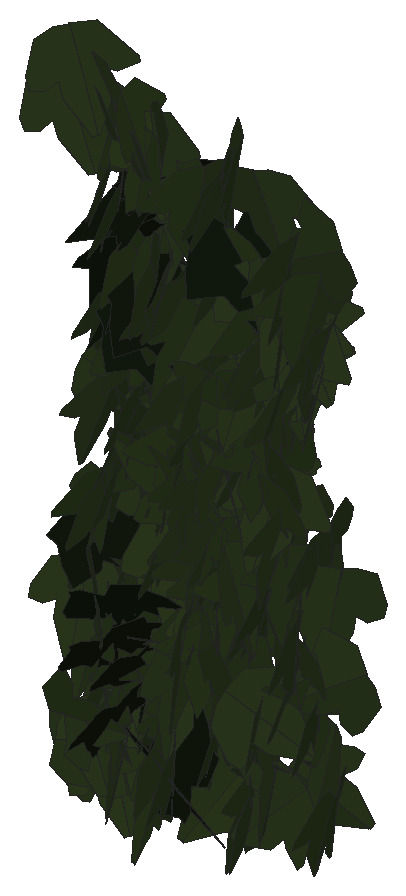
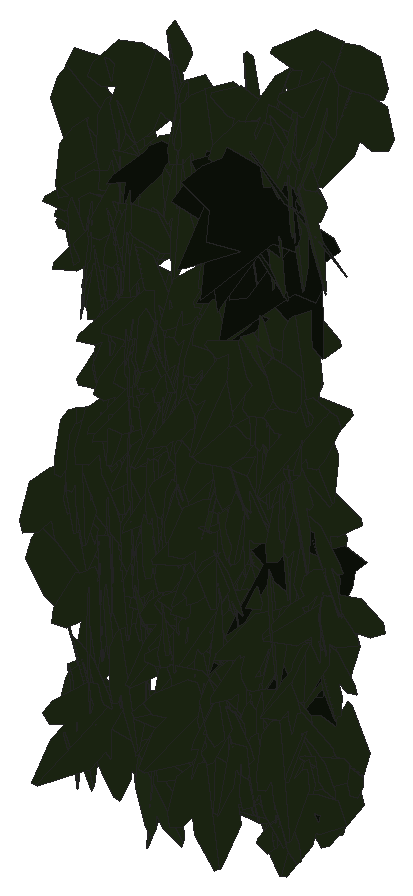
# SketchUp Ruby script. Lengths in inches.
U = 1.inch
M = Sketchup.active_model
def pt(a) = Geom::Point3d.new(a.map { |v| v * U })
def face(e, loops, mat)
  f = e.add_face(loops[0].map { |a| pt(a) })
  loops[1..].each { |l| e.add_face(l.map { |a| pt(a) }).erase! }
  f.material = f.back_material = mat if mat
  f
end
# faces: each face lists its corners as indices into pts; further lists are holes
def faces(e, pts, list, mat = nil) = list.each { |f| face(e, (f[0].is_a?(Array) ? f : [f]).map { |l| l.map { |i| pts[i] } }, mat) }
# xy, xz, yz: faces in a plane at the given z, y or x. An outline is a flat list of corners, or four numbers for a rectangle; further outlines are holes
def ring(l) = l.size == 4 ? [[l[0], l[1]], [l[2], l[1]], [l[2], l[3]], [l[0], l[3]]] : l.each_slice(2).to_a
def flat(e, list, mat, &to3) = list.each { |f| face(e, (f[0].is_a?(Array) ? f : [f]).map { |l| ring(l).map { |u, v| to3.(u, v) } }, mat) }
def xy(e, z, list, mat = nil) = flat(e, list, mat) { |x, y| [x, y, z] }
def xz(e, y, list, mat = nil) = flat(e, list, mat) { |x, z| [x, y, z] }
def yz(e, x, list, mat = nil) = flat(e, list, mat) { |y, z| [x, y, z] }
def lines(e, pts, list) = list.each { |a, b| e.add_line(pt(pts[a]), pt(pts[b])) }
# prism: a flat outline (further loops are holes) pulled along v
def prism(e, loops, v, mat = nil)
  f = face(e, loops, mat); d = Geom::Vector3d.new(v.map { |x| x * U })
  f.pushpull(f.normal.samedirection?(d) ? d.length : -d.length)
end
def box(e, o, s, mat = nil) = prism(e, [[o, [o[0] + s[0], o[1], o[2]], [o[0] + s[0], o[1] + s[1], o[2]], [o[0], o[1] + s[1], o[2]]]], [0, 0, s[2]], mat)
def at(x, y, z, deg = 0) = Geom::Transformation.translation(pt([x, y, z])) * Geom::Transformation.rotation(ORIGIN, Z_AXIS, deg.degrees)
def axes(o, x, y, z) = Geom::Transformation.new([*x, 0, *y, 0, *z, 0, *pt(o).to_a, 1])
def part(name) = M.definitions.add(name)
# library, detail: a bought-in or finely detailed component or shape, given as its bounding box
def library(name, o, s) = part(name).tap { |d| box(d.entities, o, s) }
def detail(e, o, s) = box(e.add_group.entities, o, s)
def put(e, d, t, mat = nil) = e.add_instance(d, t).tap { |i| i.material = mat if mat }
def group(e, t, mat = nil) = e.add_group.tap { |g| g.transformation = t; g.material = mat if mat }.entities
root = M.entities
M.materials.add("efeu1").color = [18, 25, 13]
M.materials.add("efeu2").color = [43, 57, 29]
c1 = part("ivyleaf_10")
p = [[0,0.5,-0.03],[-0.0625,2.02,-0.43],[-0.19,2.01,-0.46],[-0.54,1.05,-0.29],[-0.52,0.625,-0.18],[-0.83,0.76,-0.28],
  [-1.16,0.64,-0.33],[-1.15,0.33,-0.24],[-0.77,-0.39,0.02],[-0.3,-0.51,0.16],[0.04,-0.48,0.23],[-0.02,2.01,-0.4375],
  [-0.06,2.01,-0.43],[0.04,-0.49,0.23],[0.67,-0.49,0.14],[1.38,0.36,-0.2],[1.375,0.51,-0.24],[0.81,0.65,-0.19],
  [0.62,0.59,-0.15],[0.6,1.09,-0.28],[0.5,1.23,-0.31]]
faces(c1.entities,p,[[0,1,2,3,4,5,6,7,8,9,10],[11,12,0,13,14,15,16,17,18,19,20]],"efeu2")
c2 = part("ivyleaf_9")
p = [[1.54,2.16,1.25],[1.36,2.04,1.19],[-0.21,0.99,0.68],[-0.71,1.11,0.82],[-0.85,0.86,0.67],[-0.8,0.17,0.21],
  [-0.9,-0.01,0.1],[-0.67,-0.16,-0.02],[-0.08,-0.08,-0.05],[-0.03,-0.6,-0.4],[0.65,-0.88,-0.66],[0.83,-0.6,-0.49],
  [1.29,-0.42,-0.43],[1.8125,-0.07,-0.26],[1.21,0.44,0.15]]
faces(c2.entities,p,[[0,1,2,3,4,5,6,7,8,9,10,11,12,13,14]],"efeu1")
put(root,c1,axes([9.67,224.62,220.65],[0.1467,-0.41314,-0.24042],[0.0299,0.25892,-0.42669],[0.47706,0.11081,0.10067]))
put(root,c1,axes([8.58,224.6875,222.96],[0.4217,0.22163,0.15183],[0.09899,0.13451,-0.47128],[-0.24975,0.42754,0.06957]))
put(root,c1,axes([11.16,224.89,218.96],[-0.19886,-0.44425,0.11444],[0.0138,-0.13046,-0.48248],[0.45854,-0.18874,0.06415]))
put(root,c1,axes([11.23,225.09,219.62],[-0.15832,-0.24896,0.40368],[-0.07553,-0.40691,-0.28057],[0.46822,-0.14982,0.09123]))
put(root,c1,axes([9.41,224.83,221.93],[0.40818,-0.21422,0.02309],[0.03016,0.00428,-0.45145],[0.23063,0.37857,0.01817]))
put(root,c1,axes([9.81,224.63,222.27],[0.25963,-0.31984,-0.28336],[-0.10263,0.27519,-0.40465],[0.4148,0.26828,0.07725]))
put(root,c1,axes([10.75,224.69,217.39],[-0.12124,0.48435,0.02665],[-0.00457,0.02632,-0.49929],[-0.48506,-0.12131,-0.00195]))
put(root,c1,axes([9.87,224.7,214.74],[0.17093,-0.42819,-0.19347],[-0.01919,0.19935,-0.45814],[0.46948,0.16405,0.05172]))
put(root,c1,axes([8.35,224.8,214.72],[-0.10473,-0.00185,0.44101],[0.45564,0.04345,0.10053],[-0.04619,0.43282,-0.0082]))
put(root,c2,axes([9.13,224.54,216.03],[0.19407,0.39607,0.0082],[-0.01493,0.01492,-0.45191],[-0.42758,0.17925,0.0195]))
put(root,c1,axes([8.57,225,216.46],[0.1144,-0.15096,0.40973],[0.36331,-0.21494,-0.17972],[0.27501,0.34675,0.06697]))
put(root,c1,axes([8.59,224.83,216.48],[0.44025,0.14921,-0.0292],[-0.0277,-0.0116,-0.45145],[-0.16162,0.40844,-0.00216]))
put(root,c1,axes([8.47,224.71,222.43],[0.42101,0.21089,0.16816],[0.10913,0.15188,-0.46371],[-0.24666,0.42715,0.08186]))
put(root,c1,axes([10.17,224.86,221.82],[-0.17767,-0.4662,0.03308],[0.00791,-0.03838,-0.49846],[0.4673,-0.1766,0.02101]))
put(root,c2,axes([9.18,224.68,215.18],[-0.06768,0.42313,-0.08229],[0.01711,-0.07764,-0.44483],[-0.46458,-0.0645,-0.00439]))
put(root,c2,axes([9.46,224.92,214.51],[0.28678,-0.25489,0.24111],[0.18599,-0.15532,-0.38274],[0.32229,0.31644,0.00634]))
put(root,c1,axes([10.66,224.82,222.34],[0.25935,-0.42246,-0.0653],[0.00861,0.08153,-0.49323],[0.42739,0.25472,0.04957]))
put(root,c1,axes([8.68,224.88,216],[0.42862,-0.17601,0.02823],[0.02631,-0.01203,-0.45152],[0.19054,0.39762,-0.00116]))
put(root,c1,axes([11.19,224.84,218.48],[0.45715,0.17957,-0.09365],[-0.10254,0.00586,-0.48934],[-0.17464,0.46661,0.04219]))
put(root,c1,axes([10.4375,224.79,219.19],[0.13312,0.01892,-0.48158],[-0.47463,0.0919,-0.12759],[0.08369,0.49112,0.04243]))
put(root,c1,axes([11.28,224.6875,218.97],[-0.38937,0.13829,0.28155],[-0.26976,0.08139,-0.41304],[-0.16006,-0.47355,0.01123]))
put(root,c1,axes([11.65,224.94,221],[-0.15441,-0.46628,0.09347],[0.00158,-0.09878,-0.49014],[0.47556,-0.15107,0.03198]))
put(root,c1,axes([9.77,224.63,214.86],[0.0513,-0.37792,-0.32334],[0.05841,0.32738,-0.37338],[0.49392,0.00054,0.07773]))
put(root,c1,axes([11.48,224.78,216.85],[0.16866,-0.44253,-0.16036],[-0.00743,0.16782,-0.47094],[0.47064,0.16124,0.05004]))
put(root,c1,axes([11.23,225,218],[0.07446,-0.47614,0.13323],[0.02803,-0.13045,-0.48187],[0.49363,0.07923,0.00726]))
put(root,c1,axes([9.32,224.74,222.42],[-0.10805,0.41927,0.06093],[-0.00412,0.0593,-0.44816],[-0.45719,-0.09962,-0.01036]))
put(root,c1,axes([9.05,224.8,221.26],[0.16785,-0.4463,-0.15046],[-0.03289,0.14823,-0.47639],[0.46983,0.16982,0.0204]))
put(root,c1,axes([11.14,224.71,220.23],[-0.00323,-0.43689,-0.24314],[0.06248,0.24089,-0.43367],[0.49607,-0.03319,0.05303]))
put(root,c1,axes([9.9,224.91,217.93],[-0.25906,-0.00575,-0.42762],[-0.42764,-0.00034,0.25908],[-0.00327,0.49997,-0.00475]))
put(root,c1,axes([11.33,224.89,221.37],[0.0282,-0.49841,-0.02817],[-0.01488,0.02736,-0.49903],[0.49898,0.02898,-0.01329]))
put(root,c1,axes([10.76,224.82,221.03],[0.36016,-0.06913,-0.33986],[-0.31593,0.13674,-0.36262],[0.14308,0.47594,0.05482]))
put(root,c1,axes([9.93,224.96,216.17],[-0.10489,0.44599,-0.20022],[-0.06066,-0.21507,-0.44729],[-0.4851,-0.06954,0.09922]))
put(root,c2,axes([9.45,224.97,220.6],[-0.40958,0.14432,-0.16302],[0.14369,-0.08956,-0.42053],[-0.17974,-0.40047,0.0353]))
put(root,c1,axes([10.97,224.59,215.86],[0.11812,0.31878,0.36665],[0.13332,0.34158,-0.33993],[-0.4672,0.17806,-0.00431]))
put(root,c2,axes([9.06,224.66,216.47],[0.34382,0.29054,-0.06122],[-0.05464,-0.03186,-0.44811],[-0.31546,0.32218,0.0109]))
put(root,c1,axes([11.1,224.8,218.42],[-0.47018,0.16933,0.016],[-0.02026,-0.00905,-0.49951],[-0.16888,-0.47037,0.01537]))
put(root,c2,axes([9.38,224.86,221.42],[-0.39068,0.24019,0.027],[-0.02653,0.00993,-0.45156],[-0.25957,-0.36254,0.00552]))
put(root,c1,axes([11.02,224.86,222.03],[-0.48749,-0.01376,-0.1103],[0.11109,-0.0442,-0.48549],[0.00361,-0.49785,0.04615]))
put(root,c1,axes([9.32,224.74,220.8125],[0.02656,-0.42828,-0.25665],[0.08787,0.25701,-0.41979],[0.4915,-0.02281,0.08892]))
put(root,c1,axes([11.9,224.88,221.56],[-0.2256,0.00204,0.44621],[-0.44309,-0.06012,-0.22374],[0.05274,-0.49637,0.02893]))
put(root,c1,axes([10.84,224.81,219.3125],[-0.28334,0.4119,0.00766],[-0.00526,0.00568,-0.49994],[-0.41194,-0.28339,0.00111]))
put(root,c1,axes([9.65,224.95,220.21],[0.01957,-0.49961,-0.00229],[-0.00005,0.00229,-0.49999],[0.49962,0.01957,0.00004]))
put(root,c2,axes([10.6,224.92,221.28],[0.06536,-0.43431,-0.23897],[0.02007,0.24315,-0.43643],[0.4953,0.04746,0.04922]))
put(root,c1,axes([10.54,224.85,218.58],[-0.49791,-0.03979,0.0225],[-0.02257,-0.00004,-0.49949],[0.03976,-0.49841,-0.00175]))
put(root,c1,axes([9.1875,224.83,222.08],[-0.35383,0.28611,0.00606],[-0.00704,0.00139,-0.45235],[-0.30898,-0.32767,0.00337]))
put(root,c1,axes([9.85,224.99,215.81],[0.16279,0.44535,-0.15863],[-0.05178,-0.14997,-0.47416],[-0.46991,0.17081,-0.00271]))
put(root,c1,axes([11.33,224.85,221.03],[0.22017,-0.4247,-0.14543],[0.01107,0.16707,-0.47113],[0.44878,0.20424,0.08297]))
put(root,c1,axes([10.39,224.87,221.86],[0.08347,-0.47543,-0.13037],[0.00495,0.13303,-0.48195],[0.49296,0.07917,0.02692]))
put(root,c1,axes([11.17,224.95,219.91],[0.01952,-0.49885,-0.02769],[0.00394,0.02786,-0.49921],[0.4996,0.01927,0.00502]))
put(root,c1,axes([9.42,224.93,222.1],[0.44369,0.04104,0.14247],[0.14324,0.04652,-0.42814],[-0.05776,0.43055,0.03268]))
put(root,c1,axes([10.32,224.82,216.23],[-0.2992,0.10595,0.38633],[-0.38576,0.05383,-0.31352],[-0.10803,-0.48567,0.04953]))
put(root,c1,axes([9.98,224.88,219.27],[-0.1077,-0.47323,-0.12021],[0.0258,0.11741,-0.48533],[0.48758,-0.11075,-0.00087]))
put(root,c1,axes([10.36,224.89,215.3],[0.22481,-0.4226,-0.14446],[-0.03424,0.14495,-0.4773],[0.4453,0.2245,0.03623]))
put(root,c1,axes([11.07,224.89,220.48],[-0.23593,-0.42617,-0.11276],[0.07263,0.08857,-0.4867],[0.43481,-0.24604,0.02011]))
put(root,c1,axes([11.34,224.93,219.57],[-0.0264,-0.49346,-0.07616],[0.02181,0.07506,-0.49385],[0.49883,-0.0294,0.01756]))
put(root,c1,axes([10.62,225.24,217.89],[-0.00156,-0.35951,0.34749],[-0.00496,-0.34747,-0.3595],[0.49997,-0.00457,-0.00248]))
put(root,c1,axes([10.8,225.26,214.71],[0.04452,-0.13242,0.48009],[0.33447,-0.34916,-0.12733],[0.36898,0.33249,0.05749]))
put(root,c1,axes([11.38,224.99,220.3],[0.47165,0.13662,-0.09426],[-0.09351,-0.01588,-0.49092],[-0.13713,0.48071,0.01057]))
put(root,c2,axes([10.1,224.74,214.58],[-0.10758,0.11868,0.47365],[-0.28732,0.37677,-0.15967],[-0.39481,-0.30653,-0.01287]))
put(root,c1,axes([9.62,224.91,220.52],[0.27513,-0.38869,-0.1524],[-0.05347,0.14821,-0.47453],[0.41406,0.27741,0.03999]))
put(root,c1,axes([8.67,224.9,222.69],[-0.40677,0.21341,-0.04444],[0.03624,-0.02745,-0.45015],[-0.23225,-0.37806,0.0076]))
put(root,c1,axes([10.51,225.06,219.38],[-0.13753,-0.47132,0.09456],[-0.01315,-0.09463,-0.49079],[0.48053,-0.13748,0.01363]))
put(root,c1,axes([11.09,224.87,220.15],[-0.06522,-0.46595,-0.16923],[0.03089,0.16654,-0.47044],[0.49476,-0.07182,0.00707]))
put(root,c1,axes([11,224.92,220.86],[0.42008,0.26202,0.06984],[0.04411,0.06102,-0.4943],[-0.26755,0.42145,0.02815]))
put(root,c1,axes([8.73,225.08,218.6875],[-0.01959,-0.42117,0.11159],[-0.01071,-0.10696,-0.43839],[0.46927,-0.02002,-0.00535]))
put(root,c2,axes([9.17,224.96,220.71],[0.00123,0.35173,-0.26619],[0.00254,-0.25595,-0.36579],[-0.46979,-0.00047,-0.00268]))
put(root,c1,axes([9.26,225.09,218.77],[0.19305,-0.3835,0.10502],[0.05187,-0.08902,-0.44],[0.42515,0.185,0.00599]))
put(root,c1,axes([10.3,224.81,219.42],[0.03069,-0.42511,-0.26141],[0.04868,0.26321,-0.42232],[0.49668,0.00047,0.05755]))
put(root,c2,axes([9.47,224.66,216.13],[0.4351,0.15995,0.03799],[-0.0471,0.19778,-0.40037],[-0.17082,0.35288,0.20718]))
put(root,c1,axes([10.35,225.06,216.17],[-0.35039,-0.32706,0.14233],[-0.07012,-0.13246,-0.47701],[0.34973,-0.35424,0.04696]))
put(root,c2,axes([9.47,224.92,220.29],[0.10809,-0.38779,-0.29654],[-0.0523,0.29278,-0.40193],[0.48537,0.11791,0.02273]))
put(root,c1,axes([10,225.05,220],[0.24252,0.37749,-0.22064],[-0.21104,-0.11992,-0.43713],[-0.38295,0.30515,0.10116]))
put(root,c1,axes([9.91,225.05,218.43],[-0.36783,-0.32118,0.10745],[-0.03799,-0.11851,-0.48426],[0.33654,-0.36442,0.06278]))
put(root,c1,axes([8.66,224.99,217.42],[0.35257,-0.26935,-0.10453],[-0.08449,0.06311,-0.44016],[0.29877,0.3357,-0.00113]))
put(root,c1,axes([8.7,225.09,214.93],[0.38472,-0.14413,0.21202],[0.20472,-0.07504,-0.39964],[0.17549,0.40351,0.00141]))
put(root,c1,axes([10.93,224.98,217.07],[0.15772,-0.46463,-0.09613],[-0.03398,0.08998,-0.49066],[0.47325,0.16131,-0.0032]))
put(root,c1,axes([10.46,224.93,218.62],[-0.25161,0.43038,-0.03831],[0.01129,-0.03776,-0.49844],[-0.43193,-0.25169,0.00929]))
put(root,c1,axes([9.87,224.93,220.38],[0.00387,-0.47826,-0.14577],[0.03989,0.1456,-0.47666],[0.49839,-0.00793,0.03928]))
put(root,c1,axes([10.64,225.18,217.05],[-0.13861,-0.44187,0.18851],[0.02481,-0.20253,-0.45647],[0.47976,-0.11719,0.07807]))
put(root,c1,axes([10.4,224.88,221.82],[0.09556,-0.43672,-0.22393],[0.00935,0.22971,-0.44401],[0.49069,0.08067,0.05207]))
put(root,c1,axes([11.63,225.08,220.28],[0.10019,-0.4897,0.0124],[0.01504,-0.00958,-0.49968],[0.48963,0.10049,0.01281]))
put(root,c1,axes([9.9,225.14,218.66],[0.1991,-0.45163,0.07994],[0.02198,-0.07765,-0.49344],[0.45812,0.2,-0.01106]))
put(root,c1,axes([9.34,225.1,214.11],[0.36834,-0.26811,0.0332],[0.01916,-0.02907,-0.45101],[0.29098,0.34131,-0.01233]))
put(root,c1,axes([10.8125,224.98,218.71],[0.0562,-0.48016,-0.12763],[-0.00895,0.12745,-0.4834],[0.49675,0.05662,0.00573]))
put(root,c1,axes([9.48,225.05,221.17],[-0.46467,-0.06381,0.00638],[0.00847,-0.09371,-0.4417],[0.06871,-0.41997,0.09759]))
put(root,c1,axes([10.91,224.92,215.68],[0.23022,-0.39661,-0.19925],[-0.01075,0.21941,-0.44916],[0.44372,0.21109,0.0925]))
put(root,c1,axes([8.68,224.95,222.33],[-0.33006,0.30955,-0.00139],[0.00092,-0.00104,-0.4524],[-0.33432,-0.30562,0.00013]))
put(root,c1,axes([10.46,224.91,220.91],[0.07881,-0.44249,-0.21906],[0.00344,0.22232,-0.44784],[0.49374,0.06909,0.03809]))
put(root,c1,axes([10.62,225.06,218.71],[0.49853,-0.00113,-0.03825],[-0.03813,0.02777,-0.49777],[0.00325,0.49923,0.0276]))
put(root,c1,axes([11.24,224.89,220.5],[0.25227,-0.35493,-0.24574],[-0.04163,0.26329,-0.42302],[0.42968,0.23389,0.10329]))
put(root,c1,axes([8.7,225.35,214.27],[0.07627,-0.15157,0.47033],[0.31717,-0.34991,-0.1642],[0.37892,0.3234,0.04277]))
put(root,c2,axes([9.21,225.05,219.77],[0.11856,-0.37666,-0.1954],[0.00218,0.19463,-0.40458],[0.45459,0.09731,0.0529]))
put(root,c1,axes([11.33,225.07,220.25],[0.32131,-0.38017,-0.04726],[0.00173,0.06311,-0.496],[0.38309,0.31857,0.04187]))
put(root,c1,axes([8.76,224.94,217.55],[0.02758,-0.45293,-0.20999],[0.04231,0.21168,-0.451],[0.49744,0.00711,0.05001]))
put(root,c1,axes([10.05,225.16,218.1],[0.0083,-0.49268,0.08482],[-0.0046,-0.0849,-0.49272],[0.49991,0.0074,-0.00594]))
put(root,c1,axes([8.6875,225.08,221.32],[0.22037,-0.3813,-0.04882],[-0.02491,0.0409,-0.44976],[0.41416,0.20534,-0.00108]))
put(root,c1,axes([8.76,225.0625,217.65],[-0.12122,-0.48365,-0.03731],[0.00225,0.0379,-0.49856],[0.48508,-0.12104,-0.00702]))
put(root,c1,axes([10.13,225.24,217.37],[0.04746,-0.46527,0.17685],[0.04298,-0.17315,-0.46709],[0.49588,0.05954,0.02356]))
put(root,c1,axes([11.33,225.18,217.47],[-0.18455,-0.44933,0.1185],[0.00168,-0.12814,-0.4833],[0.46469,-0.17799,0.04881]))
put(root,c1,axes([11.56,225.05,219.8],[0.29363,-0.38793,-0.11529],[-0.0382,0.11523,-0.48504],[0.40289,0.29366,0.03803]))
put(root,c1,axes([9.95,225.2,218.06],[-0.06103,-0.48292,0.11431],[-0.00805,-0.11419,-0.48672],[0.4962,-0.06125,0.00617]))
put(root,c1,axes([10.83,225.15,218.99],[0.41401,-0.2799,-0.01576],[-0.01987,-0.00127,-0.4996],[0.27964,0.41431,-0.01218]))
put(root,c1,axes([9.86,225.25,215.37],[-0.05411,-0.46459,0.17672],[0.01816,-0.17949,-0.46632],[0.49673,-0.04404,0.03629]))
put(root,c1,axes([9.25,224.97,219.78],[0.41457,0.09497,0.18851],[0.14433,0.17545,-0.38994],[-0.16737,0.38655,0.13067]))
put(root,c1,axes([11.4,224.9375,220.52],[0.21001,0.42244,0.16564],[0.07592,0.14724,-0.47176],[-0.44736,0.2233,-0.0023]))
put(root,c1,axes([11.2,225.07,220.32],[0.45451,0.19228,0.08033],[0.06907,0.04285,-0.49335],[-0.19661,0.45956,0.01239]))
put(root,c1,axes([10.74,225.15,219.33],[-0.25563,0.35311,-0.24488],[0.14846,-0.19482,-0.4359],[-0.40326,-0.29556,-0.00524]))
put(root,c1,axes([9.37,225.04,219.92],[-0.37161,-0.21391,-0.16469],[0.1775,0.0328,-0.41748],[0.22608,-0.37735,0.05706]))
put(root,c1,axes([10.01,225.37,216.73],[0.11095,-0.11627,0.47347],[0.36397,-0.30331,-0.15977],[0.32437,0.38011,0.01734]))
put(root,c1,axes([10.99,225.11,219.37],[-0.30399,0.38321,-0.10364],[-0.00412,-0.13357,-0.48181],[-0.39696,-0.29207,0.08436]))
put(root,c1,axes([9.27,225.03,221.82],[-0.4263,-0.15261,-0.10466],[0.10175,0.03539,-0.44013],[0.16919,-0.40581,0.00097]))
put(root,c1,axes([9.99,225.09,215.69],[-0.3942,0.27762,-0.13242],[0.10374,-0.08263,-0.48209],[-0.28956,-0.40755,0.00754]))
put(root,c1,axes([8.73,225.09,216.1875],[0.15654,-0.03818,0.4247],[0.43324,0.1034,-0.13802],[-0.09225,0.4208,0.07245]))
put(root,c1,axes([10.52,225.24,218.03],[0.11933,0.4328,-0.22011],[-0.05,-0.2145,-0.44888],[-0.48297,0.12914,-0.00792]))
put(root,c2,axes([9.29,224.92,215.74],[0.06299,0.43016,-0.02915],[-0.01975,-0.02579,-0.4512],[-0.46514,0.05935,0.01521]))
put(root,c1,axes([9.17,225.16,220.81],[-0.39913,0.21075,-0.09436],[0.0228,-0.14005,-0.42775],[-0.24676,-0.35383,0.1131]))
put(root,c1,axes([9.45,225.33,218.16],[0.22562,-0.26815,0.2823],[0.19677,-0.20179,-0.35315],[0.36206,0.27677,0.01602]))
put(root,c1,axes([11.29,224.98,219.8],[0.10205,-0.40879,-0.26921],[-0.04827,0.26525,-0.42108],[0.48709,0.11194,0.01467]))
put(root,c1,axes([8.72,225.11,216.49],[-0.45054,-0.1109,0.05598],[-0.0558,-0.01517,-0.44892],[0.12088,-0.42035,0.00143]))
put(root,c1,axes([11.25,225.06,220.0625],[0.16661,0.46931,0.04458],[-0.02066,0.0545,-0.49659],[-0.47097,0.16363,0.03755]))
put(root,c1,axes([9.61,225.16,217.1],[0.47071,0.16678,0.02484],[0.02051,0.01649,-0.49931],[-0.16737,0.47108,0.00868]))
put(root,c1,axes([11.91,225.23,216.23],[-0.25781,0.01477,0.42815],[-0.40317,-0.17733,-0.23665],[0.14486,-0.46726,0.10335]))
put(root,c1,axes([8.47,224.93,214.44],[-0.02515,-0.1388,-0.47969],[0.42581,0.24495,-0.0932],[0.26087,-0.4132,0.10588]))
put(root,c1,axes([9.15,225.09,219.46],[-0.28321,-0.30945,-0.16346],[0.15551,0.08224,-0.41824],[0.34106,-0.29446,0.05497]))
put(root,c1,axes([11.29,225.11,215.86],[-0.35186,-0.34741,-0.07416],[0.04698,0.05795,-0.4944],[0.35212,-0.35489,-0.00814]))
put(root,c1,axes([9,225.375,215.32],[-0.0575,-0.43776,0.23464],[0.02108,-0.23815,-0.43914],[0.49624,-0.0406,0.04584]))
put(root,c1,axes([11.11,225.16,214.53],[0.36662,-0.11014,-0.32165],[-0.30949,0.0877,-0.38278],[0.14074,0.47977,-0.00387]))
put(root,c1,axes([10.42,224.89,218.49],[-0.0319,-0.29818,-0.40009],[0.12967,0.38218,-0.29517],[0.48184,-0.1226,0.05295]))
put(root,c2,axes([9.13,224.89,220.69],[0.28658,0.33495,0.08463],[0.05405,0.06417,-0.44441],[-0.36832,0.27003,0.00063]))
put(root,c1,axes([10.8125,225.11,219.85],[0.36159,-0.28896,-0.18908],[-0.10623,0.16741,-0.45901],[0.32858,0.37212,0.05968]))
put(root,c1,axes([10.35,225.26,218.33],[-0.42173,-0.09421,-0.25153],[-0.2478,-0.04416,0.43202],[-0.10362,0.48905,-0.00944]))
put(root,c1,axes([9.57,225.0625,217.23],[0.10819,-0.43754,-0.21646],[-0.03271,0.21472,-0.45036],[0.48706,0.11161,0.01784]))
put(root,c1,axes([10.59,225.18,218.45],[-0.49959,-0.01872,-0.0078],[0.01114,-0.0926,-0.49122],[0.01694,-0.49099,0.09294]))
put(root,c1,axes([8.7,225.17,219.8125],[0.02934,-0.42918,-0.06813],[-0.00865,0.06513,-0.44722],[0.4688,0.02806,-0.00399]))
put(root,c2,axes([8.65,225,217.17],[0.02937,-0.16575,-0.41731],[0.04995,0.40087,-0.16895],[0.46621,-0.03251,0.0444]))
put(root,c1,axes([11.1,225.19,218.03],[-0.20472,-0.45605,-0.01028],[0.00312,0.00987,-0.49989],[0.45616,-0.20474,-0.00119]))
put(root,c1,axes([9.15,225.1,219.4],[-0.0492,-0.39844,-0.17524],[0.06392,0.1621,-0.41528],[0.46282,-0.06475,0.03872]))
put(root,c1,axes([9.63,225.38,214.96],[-0.05239,-0.45571,0.19895],[0.00551,-0.20057,-0.45798],[0.49722,-0.04579,0.02604]))
put(root,c1,axes([9.13,225.1,218.79],[0.08411,-0.4537,-0.19258],[-0.01731,0.19252,-0.46112],[0.49257,0.08423,0.01668]))
put(root,c1,axes([8.89,225.11,217.8],[0.13103,-0.44424,-0.18837],[-0.02275,0.18929,-0.46223],[0.48199,0.1297,0.02939]))
put(root,c1,axes([9.39,225.2,220.2],[0.41446,0.18581,-0.08963],[-0.11192,0.01826,-0.43896],[-0.19081,0.3929,0.06279]))
put(root,c1,axes([10.82,225.13,218.52],[-0.44387,0.22852,-0.02764],[0.019,-0.02346,-0.49909],[-0.2294,-0.44411,0.01214]))
put(root,c1,axes([10.27,225.16,216.45],[-0.24452,-0.41841,-0.12304],[0.11736,0.07272,-0.48056],[0.42004,-0.2639,0.06265]))
put(root,c1,axes([11.24,225.1,216.48],[-0.41461,0.11529,0.25458],[-0.25037,0.04914,-0.43],[-0.12417,-0.48404,0.01698]))
put(root,c1,axes([9.83,225.3,215.76],[0.0009,-0.49762,0.0487],[-0.00581,-0.0487,-0.49759],[0.49997,0.00033,-0.00587]))
put(root,c1,axes([9.64,225.5,215.44],[-0.11029,-0.32573,0.36295],[-0.05441,-0.36158,-0.34103],[0.48464,-0.11472,0.04431]))
put(root,c1,axes([9.96,225.1875,217.46],[-0.1547,-0.46892,-0.07862],[0.02445,0.07473,-0.49378],[0.47484,-0.15662,-0.00019]))
put(root,c1,axes([9.4,225.07,220.58],[0.03823,0.41081,0.14413],[-0.06439,0.14234,-0.42298],[-0.46379,0.0141,0.07061]))
put(root,c1,axes([9.36,225.21,219.18],[-0.08718,0.42449,-0.05214],[0.00376,-0.05036,-0.44934],[-0.46162,-0.08058,0.00619]))
put(root,c1,axes([10.91,225.16,219.09],[0.14768,-0.4434,-0.17773],[-0.00121,0.18569,-0.46424],[0.47769,0.13755,0.05377]))
put(root,c1,axes([8.7,225.18,214.23],[0.3373,0.28694,0.10055],[0.07099,0.07133,-0.44101],[-0.31921,0.31906,0.00817]))
put(root,c1,axes([10.35,225.18,218.92],[-0.44313,-0.2106,-0.09636],[0.09067,0.03366,-0.49056],[0.21311,-0.45223,0.00836]))
put(root,c1,axes([10.52,225.09,219.45],[0.23048,0.42904,0.11315],[-0.05883,0.15592,-0.47141],[-0.43979,0.20399,0.12236]))
put(root,c2,axes([9.54,225.02,221.21],[0.19335,0.39618,-0.01525],[-0.00883,-0.0124,-0.45214],[-0.42808,0.1792,0.00244]))
put(root,c1,axes([9.69,225.18,215.91],[-0.03867,-0.47595,-0.14824],[0.00355,0.14842,-0.47745],[0.49849,-0.03798,-0.0081]))
put(root,c1,axes([11.56,225.3,214.62],[0.11577,-0.48569,-0.0265],[-0.00458,0.02615,-0.49929],[0.48639,0.11585,0.00161]))
put(root,c1,axes([9.4,225.28,217.54],[0.45922,0.0671,-0.06517],[-0.07289,0.02719,-0.44603],[-0.06721,0.42893,0.03846]))
put(root,c1,axes([11.48,225.16,220.25],[0.2325,-0.40137,-0.18666],[0.02558,0.22267,-0.44695],[0.44191,0.19828,0.12408]))
put(root,c1,axes([8.89,225.16,218.56],[-0.38173,0.23169,0.10717],[-0.09478,0.05408,-0.43951],[-0.25693,-0.36417,0.00291]))
put(root,c1,axes([9.61,225.27,216.17],[-0.3358,-0.36972,-0.0234],[0.0361,-0.00123,-0.49869],[0.36869,-0.33661,0.02752]))
put(root,c1,axes([8.78,225.12,214.875],[-0.2511,0.33931,0.1472],[-0.08649,0.11671,-0.42778],[-0.38753,-0.24591,0.00009]))
put(root,c1,axes([10.62,225.22,218.35],[0.13717,0.48065,0.01281],[-0.00658,0.0152,-0.49973],[-0.48077,0.13692,0.01049]))
put(root,c1,axes([9.97,225.35,217.05],[-0.17237,-0.46517,0.06245],[-0.03055,-0.05527,-0.496],[0.46835,-0.17481,-0.00937]))
put(root,c1,axes([9.9375,225.35,216.71],[0.44306,0.12122,-0.19749],[-0.193,-0.0428,-0.45926],[-0.12825,0.48319,0.00887]))
put(root,c1,axes([9.33,225.32,215.05],[0.18475,-0.46196,-0.04963],[-0.01193,0.04867,-0.49748],[0.46446,0.18501,0.00697]))
put(root,c1,axes([9.96,225.25,217.82],[-0.4854,0.06406,0.10142],[-0.10617,-0.03264,-0.48751],[-0.05583,-0.4948,0.04529]))
put(root,c1,axes([10.72,225.22,218.42],[0.0876,0.49173,0.02292],[0.01039,0.02143,-0.49943],[-0.49216,0.08798,-0.00646]))
put(root,c1,axes([9.37,225.26,219.85],[-0.41888,-0.19673,0.01003],[-0.0119,0.0004,-0.45225],[0.21239,-0.38797,-0.00556]))
put(root,c1,axes([10,225.24,218.58],[0.02836,0.49911,-0.0093],[-0.00004,-0.00931,-0.49991],[-0.4992,0.02836,-0.00049]))
put(root,c1,axes([10.96,225.14,219.29],[0.03348,0.47999,0.13596],[0.00919,0.13565,-0.48116],[-0.49879,0.03472,0.00026]))
put(root,c1,axes([9.32,225.44,218.34],[-0.04633,-0.40769,0.15134],[-0.00917,-0.14541,-0.42629],[0.46742,-0.04326,0.00664]))
put(root,c1,axes([8.71,225.25,218.1],[0.17447,-0.37345,-0.15999],[-0.06945,0.13979,-0.42315],[0.43064,0.17384,-0.00343]))
put(root,c1,axes([10.33,225.29,217.58],[0.00562,0.49445,-0.07406],[-0.00292,-0.07403,-0.49448],[-0.49996,0.00599,0.00206]))
put(root,c1,axes([8.52,224.98,216.66],[-0.02887,-0.05689,-0.44765],[0.16116,0.40377,-0.06514],[0.44035,-0.15151,-0.00551]))
put(root,c1,axes([10.19,225.28,217.4],[0.06378,-0.48544,-0.10141],[0.00979,0.10346,-0.48908],[0.49582,0.0604,0.0227]))
put(root,c1,axes([10.24,225.35,214.43],[0.41914,0.09034,-0.25722],[-0.25876,-0.01667,-0.42751],[-0.08582,0.49149,0.03277]))
put(root,c1,axes([11.44,225.39,215.1875],[0.41412,-0.27781,0.0364],[0.03686,-0.01038,-0.49853],[0.27775,0.41559,0.01188]))
put(root,c1,axes([9.66,225.34,218.68],[0.46383,0.05532,-0.04308],[-0.04604,0.00687,-0.45017],[-0.05874,0.43141,0.01269]))
put(root,c1,axes([9.42,225.41,217.68],[0.10659,-0.4186,0.06787],[0.03769,-0.05875,-0.44678],[0.45599,0.10271,0.02106]))
put(root,c1,axes([11.58,225.42,217.15],[-0.33178,-0.36029,0.10054],[0.01273,-0.14519,-0.47829],[0.37384,-0.31482,0.10552]))
put(root,c1,axes([9.375,225.36,215.59],[-0.44083,0.14657,-0.18491],[0.14391,-0.14349,-0.45684],[-0.18698,-0.45599,0.08432]))
put(root,c1,axes([9.96,225.31,216.41],[-0.41526,-0.2783,0.01063],[-0.009,-0.00567,-0.49989],[0.27835,-0.41535,-0.0003]))
put(root,c1,axes([8.78,225.23,214.01],[0.04982,0.42976,-0.05095],[-0.01763,0.05096,0.44896],[0.46682,-0.04394,0.02239]))
put(root,c1,axes([9.3,225.33,219.29],[0.12122,0.41543,-0.06613],[-0.06454,-0.04937,-0.44516],[-0.44928,0.11918,0.0461]))
put(root,c1,axes([10.76,225.19,218.7],[-0.19689,-0.39651,-0.23241],[0.09206,0.21368,-0.44256],[0.45029,-0.21706,-0.01114]))
put(root,c1,axes([9.48,225.28,219.35],[-0.0885,0.42696,0.01515],[-0.02014,0.01125,-0.45183],[-0.46095,-0.08247,0.01683]))
put(root,c1,axes([10.56,225.16,214.26],[0.13863,-0.36904,-0.30756],[-0.03331,0.31195,-0.38933],[0.47924,0.12844,0.06191]))
put(root,c1,axes([11.0625,225.33,215.83],[0.17678,-0.45679,-0.10046],[-0.00923,0.10397,-0.48898],[0.46762,0.17474,0.02832]))
put(root,c1,axes([10.31,225.29,217.66],[-0.45366,0.04093,0.2062],[-0.20743,-0.00746,-0.45488],[-0.03416,-0.49827,0.02374]))
put(root,c1,axes([9.23,225.32,218.01],[-0.169,-0.39002,-0.11685],[0.10373,0.08142,-0.43303],[0.4259,-0.17459,0.0591]))
put(root,c1,axes([9.83,225.3125,216.82],[0.22471,-0.41758,-0.15854],[-0.02545,0.16521,-0.47123],[0.44594,0.21985,0.05299]))
put(root,c1,axes([9.33,225.42,215.59],[-0.18388,-0.4629,0.04367],[-0.02632,-0.03653,-0.49797],[0.46421,-0.18543,-0.01093]))
put(root,c1,axes([9.16,225.25,214.68],[0.27635,-0.2391,-0.26836],[-0.14298,0.23017,-0.35834],[0.35199,0.28121,0.06514]))
put(root,c1,axes([11.61,225.3,214.68],[0.23985,-0.40056,-0.17897],[-0.03669,0.18494,-0.46309],[0.43718,0.23527,0.05933]))
put(root,c1,axes([11.375,225.27,215.65],[0.1697,-0.41861,-0.21441],[-0.02572,0.21933,-0.44859],[0.46962,0.16328,0.0529]))
put(root,c1,axes([9.4,225.29,218.3],[-0.34702,-0.12961,-0.27355],[0.27369,0.07357,-0.35966],[0.15933,-0.40867,0.02201]))
put(root,c1,axes([10.46,225.35,217.63],[0.14178,-0.46439,-0.11934],[-0.00035,0.12435,-0.48429],[0.47948,0.13741,0.03494]))
put(root,c1,axes([11.43,225.34,217.64],[0.07631,-0.47454,-0.1378],[0.00095,0.13957,-0.48012],[0.49414,0.07301,0.0222]))
put(root,c1,axes([10.17,225.4,216.81],[-0.32564,-0.3794,0.00343],[0.00313,-0.00721,-0.49994],[0.3794,-0.32558,0.00707]))
put(root,c1,axes([9.84,225.47,216.25],[-0.15096,-0.4745,0.0454],[0.02941,-0.05681,-0.49589],[0.47576,-0.14705,0.04506]))
put(root,c1,axes([10.1875,225.27,217.3],[0.28822,-0.21508,-0.34737],[-0.23383,0.26177,-0.35609],[0.33504,0.36772,0.05031]))
put(root,c1,axes([9.65,225.34,216.86],[-0.49785,0.03744,0.02721],[-0.02731,-0.00028,-0.49925],[-0.03737,-0.4986,0.00233]))
put(root,c2,axes([9.27,225.07,221.28],[0.31807,0.26566,0.1858],[0.0593,0.19723,-0.39916],[-0.34063,0.2824,0.104]))
put(root,c1,axes([10.39,225.43,217.08],[0.10388,-0.48619,-0.05319],[-0.00973,0.05231,-0.49716],[0.48899,0.10432,0.00141]))
put(root,c1,axes([10.34,225.6,214.26],[0.14338,-0.44437,0.17882],[0.05406,-0.17046,-0.46693],[0.47594,0.15324,-0.00084]))
put(root,c1,axes([9.05,225.39,216],[0.04659,0.49554,-0.04767],[-0.04044,-0.04396,-0.49642],[-0.49618,0.05011,0.03599]))
put(root,c1,axes([9.36,225.4375,216.53],[0.40166,0.22403,-0.02796],[-0.02692,-0.01074,-0.45152],[-0.2422,0.37272,0.0038]))
put(root,c1,axes([8.87,225.49,214.95],[-0.0533,-0.49537,0.04205],[-0.00214,-0.04206,-0.49822],[0.49715,-0.05329,0.00236]))
put(root,c1,axes([8.87,225.39,216.81],[0.19367,-0.44394,-0.12412],[0.00186,0.13538,-0.48132],[0.46096,0.18598,0.05409]))
put(root,c1,axes([9.71,225.46,216.17],[0.28632,0.4028,-0.076],[-0.04309,-0.06262,-0.49419],[-0.40763,0.28954,-0.00115]))
put(root,c1,axes([9.48,225.4,217.63],[-0.45985,0.04829,0.07784],[-0.08479,-0.03084,-0.44381],[-0.04544,-0.43121,0.04046]))
put(root,c1,axes([9.38,225.46,216.7],[-0.39887,-0.14879,0.18218],[-0.16998,-0.07788,-0.4139],[0.18089,-0.40128,0.01278]))
put(root,c1,axes([9.11,225.45,215.42],[0.41745,0.27469,-0.01686],[-0.01492,-0.00799,-0.49971],[-0.2748,0.41771,0.00153]))
put(root,c1,axes([11.49,225.37,217.79],[0.02472,-0.47567,-0.15207],[-0.00181,0.15217,-0.47628],[0.49939,0.0241,0.0058]))
put(root,c1,axes([10.95,225.37,214.45],[0.09881,0.14729,-0.46749],[-0.47595,0.14276,-0.05562],[0.1171,0.45599,0.16841]))
put(root,c1,axes([9.66,225.47,215.92],[0.49055,-0.09524,-0.0171],[-0.00738,0.05129,-0.49731],[0.09648,0.48816,0.04891]))
put(root,c1,axes([10,225.36,216.41],[0.10642,-0.45195,-0.18551],[-0.00922,0.18797,-0.46323],[0.48846,0.10201,0.03167]))
put(root,c1,axes([8.73,225.12,215.78],[0.05483,-0.02638,-0.44847],[0.02089,0.43389,-0.02524],[0.46612,-0.01634,0.05388]))
put(root,c1,axes([9.31,225.625,215.62],[-0.06706,-0.38312,0.20431],[-0.0305,-0.19443,-0.40363],[0.46399,-0.06815,0.00299]))
put(root,c1,axes([9.47,225.57,217.06],[0.3512,-0.26673,0.11549],[0.09708,-0.0655,-0.43736],[0.29655,0.33733,0.0064]))
put(root,c1,axes([8.9,225.375,216.42],[0.08546,0.49026,0.04842],[-0.00213,0.04951,-0.49754],[-0.49264,0.08483,0.01055]))
put(root,c2,axes([9.23,225.19,221.38],[0.26761,0.35206,0.0648],[0.03404,0.05401,-0.4477],[-0.38463,0.24973,0.00547]))
put(root,c1,axes([8.52,225.19,218.83],[0.08161,0.28509,0.33254],[0.027,0.3212,-0.30398],[-0.46187,0.06915,0.04099]))
put(root,c1,axes([10.73,225.4,217.81],[0.18257,-0.43537,-0.16469],[-0.00735,0.17419,-0.46862],[0.46542,0.17353,0.0572]))
put(root,c1,axes([9.41,225.46,215.67],[-0.41625,-0.25611,-0.10558],[0.13013,-0.01253,-0.48261],[0.24455,-0.42924,0.07709]))
put(root,c1,axes([10.76,225.48,215.47],[0.08395,-0.48656,-0.07882],[-0.01768,0.07693,-0.49373],[0.49258,0.08569,-0.00429]))
put(root,c1,axes([10.54,225.4,216.66],[0.09988,-0.4514,-0.19042],[-0.01478,0.19147,-0.46165],[0.4897,0.09785,0.0249]))
put(root,c1,axes([10.53,225.53,216.54],[0.20802,-0.45348,-0.033],[-0.00727,0.03297,-0.49886],[0.45462,0.20802,0.00712]))
put(root,c1,axes([11.15,225.39,216.4],[0.19494,-0.40594,-0.21729],[-0.04139,0.21955,-0.44731],[0.45857,0.19239,0.052]))
put(root,c1,axes([9.47,225.51,217.01],[0.05756,0.4254,-0.07658],[-0.05911,-0.06693,-0.44337],[-0.4625,0.0615,0.04713]))
put(root,c1,axes([8.66,225.5,215.15],[-0.01482,-0.49234,-0.08593],[-0.01099,0.08627,-0.49238],[0.49966,-0.0127,-0.01338]))
put(root,c1,axes([10.09,225.54,216.31],[0.1469,-0.47027,-0.08526],[-0.00427,0.08791,-0.49219],[0.47791,0.14533,0.02181]))
put(root,c1,axes([9.55,225.6,217.3125],[0.29788,0.33331,-0.04719],[-0.03316,-0.03349,-0.44993],[-0.36177,0.27751,0.00238]))
put(root,c1,axes([9.61,225.5,215.9],[0.31711,0.36428,0.12938],[0.07422,0.10686,-0.48278],[-0.37938,0.32539,0.01369]))
put(root,c1,axes([9.64,225.52,217.875],[-0.33006,0.30708,0.04063],[-0.0256,0.03153,-0.45054],[-0.33334,-0.30648,-0.00564]))
put(root,c1,axes([9.46,225.62,217.56],[-0.31161,-0.32532,-0.01233],[0.00842,0.00894,-0.45223],[0.35148,-0.28864,-0.0001]))
put(root,c1,axes([9.3,225.48,218.625],[-0.00079,-0.34796,0.27149],[0.00046,0.26105,0.36188],[-0.4698,0.00084,-0.0001]))
put(root,c1,axes([9.9375,225.44,216.27],[-0.14996,-0.32414,-0.34993],[0.22554,0.27503,-0.35141],[0.42029,-0.26324,0.06372]))
put(root,c1,axes([11.07,225.49,214.66],[-0.24589,-0.27585,-0.33682],[0.27487,0.20162,-0.36578],[0.33762,-0.36504,0.05249]))
put(root,c1,axes([9.62,225.4,216.25],[0.17991,0.30876,0.34972],[0.06895,0.35311,-0.34722],[-0.46139,0.17316,0.08448]))
put(root,c1,axes([9.81,225.36,216.62],[0.07949,-0.10045,0.48331],[-0.24685,0.41584,0.12703],[-0.42749,-0.25881,0.01652]))
put(root,c1,axes([9.3,225.82,216.66],[-0.23085,0.33203,-0.18975],[0.00209,-0.20853,-0.39703],[-0.40916,-0.1884,0.10503]))
put(root,c1,axes([9.54,225.57,215.29],[-0.24115,0.42213,0.11685],[-0.05691,0.10206,-0.48615],[-0.43429,-0.24778,-0.00118]))
put(root,c1,axes([9.21,225.69,215.24],[0.3087,-0.27872,-0.17966],[-0.12314,0.1304,-0.41499],[0.33205,0.30747,0.01314]))
put(root,c1,axes([9.46,225.56,216.57],[0.18343,0.33124,0.23408],[0.08607,0.21164,-0.38646],[-0.42386,0.18632,0.02283]))
put(root,c1,axes([9.24,225.73,215.18],[-0.4223,0.18791,0.03318],[-0.04542,-0.01403,-0.45004],[-0.20077,-0.39207,0.03201]))
put(root,c1,axes([9.38,225.85,214.57],[-0.2295,-0.3785,0.0296],[-0.00938,-0.02776,-0.45139],[0.40982,-0.21259,0.00624]))
put(root,c1,axes([9.48,225.81,215.48],[-0.2283,-0.01276,-0.39517],[0.40842,-0.05183,-0.21699],[-0.04229,-0.43171,0.03773]))
put(root,c1,axes([8.67,225.82,219.74],[0.37407,0.13719,0.23357],[0.21511,0.10599,-0.38679],[-0.18577,0.39896,0.02244]))
put(root,c1,axes([9.49,225.8125,215.39],[-0.30974,-0.17594,-0.28674],[0.26415,0.12808,-0.3496],[0.23451,-0.37665,0.01506]))
put(root,c1,axes([8.68,225.8,219.6],[0.18924,-0.32344,0.24146],[-0.12653,0.20055,0.38252],[-0.41096,-0.21069,-0.00659]))
put(root,c1,axes([9.06,225.89,219.54],[-0.07288,-0.37342,-0.22118],[0.16749,0.17961,-0.37916],[0.43284,-0.13238,0.10948]))
